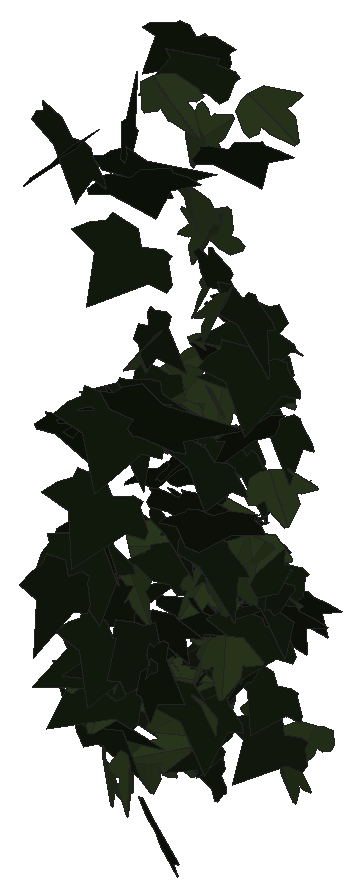
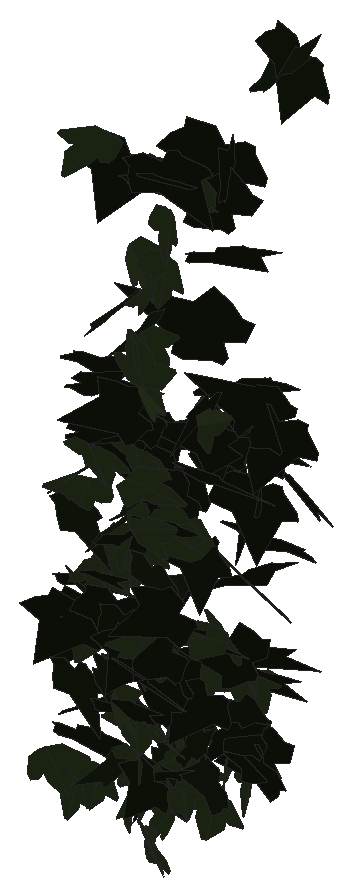
# SketchUp Ruby script. Lengths in inches.
U = 1.inch
M = Sketchup.active_model
def pt(a) = Geom::Point3d.new(a.map { |v| v * U })
def face(e, loops, mat)
  f = e.add_face(loops[0].map { |a| pt(a) })
  loops[1..].each { |l| e.add_face(l.map { |a| pt(a) }).erase! }
  f.material = f.back_material = mat if mat
  f
end
# faces: each face lists its corners as indices into pts; further lists are holes
def faces(e, pts, list, mat = nil) = list.each { |f| face(e, (f[0].is_a?(Array) ? f : [f]).map { |l| l.map { |i| pts[i] } }, mat) }
# xy, xz, yz: faces in a plane at the given z, y or x. An outline is a flat list of corners, or four numbers for a rectangle; further outlines are holes
def ring(l) = l.size == 4 ? [[l[0], l[1]], [l[2], l[1]], [l[2], l[3]], [l[0], l[3]]] : l.each_slice(2).to_a
def flat(e, list, mat, &to3) = list.each { |f| face(e, (f[0].is_a?(Array) ? f : [f]).map { |l| ring(l).map { |u, v| to3.(u, v) } }, mat) }
def xy(e, z, list, mat = nil) = flat(e, list, mat) { |x, y| [x, y, z] }
def xz(e, y, list, mat = nil) = flat(e, list, mat) { |x, z| [x, y, z] }
def yz(e, x, list, mat = nil) = flat(e, list, mat) { |y, z| [x, y, z] }
def lines(e, pts, list) = list.each { |a, b| e.add_line(pt(pts[a]), pt(pts[b])) }
# prism: a flat outline (further loops are holes) pulled along v
def prism(e, loops, v, mat = nil)
  f = face(e, loops, mat); d = Geom::Vector3d.new(v.map { |x| x * U })
  f.pushpull(f.normal.samedirection?(d) ? d.length : -d.length)
end
def box(e, o, s, mat = nil) = prism(e, [[o, [o[0] + s[0], o[1], o[2]], [o[0] + s[0], o[1] + s[1], o[2]], [o[0], o[1] + s[1], o[2]]]], [0, 0, s[2]], mat)
def at(x, y, z, deg = 0) = Geom::Transformation.translation(pt([x, y, z])) * Geom::Transformation.rotation(ORIGIN, Z_AXIS, deg.degrees)
def axes(o, x, y, z) = Geom::Transformation.new([*x, 0, *y, 0, *z, 0, *pt(o).to_a, 1])
def part(name) = M.definitions.add(name)
# library, detail: a bought-in or finely detailed component or shape, given as its bounding box
def library(name, o, s) = part(name).tap { |d| box(d.entities, o, s) }
def detail(e, o, s) = box(e.add_group.entities, o, s)
def put(e, d, t, mat = nil) = e.add_instance(d, t).tap { |i| i.material = mat if mat }
def group(e, t, mat = nil) = e.add_group.tap { |g| g.transformation = t; g.material = mat if mat }.entities
root = M.entities
M.materials.add("1026 AP 7946 SUNNY SIDE UP").color = [254, 231, 186]
M.materials.add("efeu1").color = [18, 25, 13]
M.materials.add("efeu2").color = [43, 57, 29]
c1 = part("ivyleaf_9")
p = [[1.54,2.16,1.25],[1.36,2.04,1.19],[-0.21,0.99,0.68],[-0.71,1.11,0.82],[-0.85,0.86,0.67],[-0.8,0.17,0.21],
  [-0.9,-0.01,0.1],[-0.67,-0.16,-0.02],[-0.08,-0.08,-0.05],[-0.03,-0.6,-0.4],[0.65,-0.88,-0.66],[0.83,-0.6,-0.49],
  [1.29,-0.42,-0.43],[1.8125,-0.07,-0.26],[1.21,0.44,0.15]]
faces(c1.entities,p,[[0,1,2,3,4,5,6,7,8,9,10,11,12,13,14]],"efeu1")
c2 = part("ivyleaf_10")
p = [[0,0.5,-0.03],[-0.0625,2.02,-0.43],[-0.19,2.01,-0.46],[-0.54,1.05,-0.29],[-0.52,0.625,-0.18],[-0.83,0.76,-0.28],
  [-1.16,0.64,-0.33],[-1.15,0.33,-0.24],[-0.77,-0.39,0.02],[-0.3,-0.51,0.16],[0.04,-0.48,0.23],[-0.02,2.01,-0.4375],
  [-0.06,2.01,-0.43],[0.04,-0.49,0.23],[0.67,-0.49,0.14],[1.38,0.36,-0.2],[1.375,0.51,-0.24],[0.81,0.65,-0.19],
  [0.62,0.59,-0.15],[0.6,1.09,-0.28],[0.5,1.23,-0.31]]
faces(c2.entities,p,[[0,1,2,3,4,5,6,7,8,9,10],[11,12,0,13,14,15,16,17,18,19,20]],"efeu2")
put(root,c1,axes([98.38,212.04,285.3],[-0.42534,0.09276,0.15739],[-0.27682,-0.04193,-0.27204],[-0.09708,-0.28684,0.08616]),"1026 AP 7946 SUNNY SIDE UP")
put(root,c1,axes([97.67,211.22,280.16],[-0.05565,-0.06134,-0.33985],[0.53891,0.05005,-0.04487],[0.09666,-0.31438,0.0545]),"1026 AP 7946 SUNNY SIDE UP")
put(root,c1,axes([97.57,211.11,280.16],[0.2723,-0.09417,0.2796],[0.37212,-0.14442,-0.20097],[0.29237,0.27152,-0.0046]),"1026 AP 7946 SUNNY SIDE UP")
put(root,c1,axes([97.9,212.59,280.82],[-0.0867,-0.10997,0.27516],[0.03381,-0.26345,-0.11947],[0.4756,-0.00132,0.05865]),"1026 AP 7946 SUNNY SIDE UP")
put(root,c1,axes([97.82,213.23,282.9],[0.4772,-0.04186,-0.00935],[-0.0204,-0.02537,-0.30326],[0.06947,0.28008,-0.02484]),"1026 AP 7946 SUNNY SIDE UP")
put(root,c2,axes([97.74,212.82,284.58],[-0.21631,-0.05215,0.29035],[0.38492,0.15206,0.14712],[-0.26962,0.25892,-0.02291]),"1026 AP 7946 SUNNY SIDE UP")
put(root,c1,axes([98.28,212.81,290.96],[0.17054,0.12703,-0.30451],[-0.26676,-0.23939,-0.17622],[-0.45956,0.1861,-0.01071]),"1026 AP 7946 SUNNY SIDE UP")
put(root,c1,axes([97.82,211.32,281.89],[0.05548,0.0684,0.35201],[0.47133,0.17878,-0.06705],[-0.3181,0.27683,-0.03796]),"1026 AP 7946 SUNNY SIDE UP")
put(root,c1,axes([98.17,212.1,284.02],[0.11313,0.29038,-0.01214],[0.00712,-0.01647,-0.31908],[-0.49355,0.06632,-0.00739]),"1026 AP 7946 SUNNY SIDE UP")
put(root,c1,axes([98.08,211.8,279.93],[-0.09047,0.25353,-0.13791],[-0.12801,0.11717,0.27492],[0.46813,0.08104,0.04852]),"1026 AP 7946 SUNNY SIDE UP")
put(root,c2,axes([98.42,213.16,284.79],[-0.2338,0.04398,-0.27004],[-0.35977,0.14226,0.15209],[0.24559,0.25028,-0.03427]),"1026 AP 7946 SUNNY SIDE UP")
put(root,c1,axes([98.05,210.36,285.49],[0.49043,0.19126,-0.1099],[-0.12411,-0.07954,-0.37108],[-0.34909,0.29697,-0.02246]),"1026 AP 7946 SUNNY SIDE UP")
put(root,c2,axes([97.74,212.98,285.03],[0.2767,0.02598,0.27299],[0.4345,-0.01331,-0.17413],[-0.00466,0.30206,-0.02689]),"1026 AP 7946 SUNNY SIDE UP")
put(root,c1,axes([97.94,211.39,280.71],[0.06599,-0.21099,-0.23244],[-0.0259,0.21449,-0.22598],[0.50994,0.0382,0.0186]),"1026 AP 7946 SUNNY SIDE UP")
put(root,c1,axes([97.86,213.04,283.46],[0.38777,0.11533,0.1459],[0.2122,0.05124,-0.27306],[-0.21364,0.26023,-0.00641]),"1026 AP 7946 SUNNY SIDE UP")
put(root,c1,axes([98.22,213.09,284.92],[-0.45097,-0.12442,-0.02544],[0.06144,-0.02551,-0.31172],[0.20555,-0.26536,0.03735]),"1026 AP 7946 SUNNY SIDE UP")
put(root,c1,axes([97.89,211.09,280.59],[0.1587,0.29361,-0.07654],[0.0097,0.0771,0.33043],[0.51447,-0.09203,0.01738]),"1026 AP 7946 SUNNY SIDE UP")
put(root,c2,axes([98.1875,211.97,286.16],[-0.10391,0.08457,-0.30816],[-0.14064,-0.28821,-0.07554],[-0.49134,0.06461,0.08679]),"1026 AP 7946 SUNNY SIDE UP")
put(root,c1,axes([98.4,210.71,281.51],[-0.43874,-0.14077,0.19038],[-0.2317,-0.12222,-0.31443],[0.31054,-0.29007,0.03437]),"1026 AP 7946 SUNNY SIDE UP")
put(root,c2,axes([98.24,210.84,279.62],[-0.30541,0.25759,0.06524],[-0.11552,0.02207,-0.33298],[-0.43291,-0.18761,0.04283]),"1026 AP 7946 SUNNY SIDE UP")
put(root,c2,axes([98.12,213.28,289.1],[0.1476,-0.01866,-0.31434],[0.11735,0.29866,0.00577],[0.48503,-0.06658,0.09426]),"1026 AP 7946 SUNNY SIDE UP")
put(root,c2,axes([98.41,213.26,285.63],[0.20047,0.11119,-0.25724],[-0.36063,-0.11983,-0.17179],[-0.27195,0.24087,0.03819]),"1026 AP 7946 SUNNY SIDE UP")
put(root,c2,axes([97.86,212.15,282.62],[0.11133,-0.03432,-0.30863],[0.4711,0.09268,0.05716],[0.14214,-0.28029,0.05229]),"1026 AP 7946 SUNNY SIDE UP")
put(root,c1,axes([98.09,212.06,281.53],[0.48351,0.07693,-0.06155],[-0.08092,-0.04655,-0.31466],[-0.14272,0.28702,-0.03013]),"1026 AP 7946 SUNNY SIDE UP")
put(root,c1,axes([98.21,213.17,280.51],[0.13488,0.21504,0.17202],[0.11905,0.1421,-0.24302],[-0.43693,0.1051,-0.01311]),"1026 AP 7946 SUNNY SIDE UP")
put(root,c2,axes([98.26,211.66,279.46],[-0.48743,0.0251,-0.01062],[0.01287,-0.03031,-0.30738],[-0.04419,-0.28572,0.02761]),"1026 AP 7946 SUNNY SIDE UP")
put(root,c1,axes([98.18,211.9,286.48],[0.17429,-0.15766,-0.26731],[-0.22103,0.21067,-0.19845],[0.44664,0.16578,0.0061]),"1026 AP 7946 SUNNY SIDE UP")
put(root,c2,axes([98.41,211.76,280.7],[0.19147,-0.02456,0.28268],[-0.28092,0.21811,0.10032],[-0.35244,-0.18719,0.0736]),"1026 AP 7946 SUNNY SIDE UP")
put(root,c1,axes([98.62,212.22,282.52],[-0.41568,-0.0099,0.16834],[-0.26152,-0.04691,-0.26046],[0.05703,-0.28728,0.0326]),"1026 AP 7946 SUNNY SIDE UP")
put(root,c2,axes([98.28,213.125,279.41],[0.208,-0.23771,0.07003],[0.04232,-0.0642,-0.2871],[0.41781,0.12484,-0.00578]),"1026 AP 7946 SUNNY SIDE UP")
put(root,c2,axes([98.04,211.61,282.33],[0.30397,-0.06339,0.24508],[0.35983,-0.08901,-0.20441],[0.18495,0.27736,-0.00511]),"1026 AP 7946 SUNNY SIDE UP")
put(root,c1,axes([98.53,210.64,281.14],[-0.52435,-0.14158,0.07959],[-0.07607,-0.08265,-0.36011],[0.2621,-0.30722,0.0547]),"1026 AP 7946 SUNNY SIDE UP")
put(root,c1,axes([98.6,212.85,290.6],[-0.51653,-0.07383,0.09281],[-0.12357,-0.06758,-0.3324],[0.15026,-0.30936,0.0457]),"1026 AP 7946 SUNNY SIDE UP")
put(root,c2,axes([98.52,210.6,281.59],[0.20623,-0.15301,-0.30995],[-0.20112,0.26508,-0.20092],[0.515,0.16479,0.04565]),"1026 AP 7946 SUNNY SIDE UP")
put(root,c1,axes([98.4,211.12,289.92],[-0.00384,-0.13812,0.34401],[0.19076,0.30589,0.14508],[-0.56521,0.10418,0.04663]),"1026 AP 7946 SUNNY SIDE UP")
put(root,c2,axes([98.31,213.03,282.66],[0.45847,0.10416,-0.01682],[-0.00974,-0.03233,-0.30889],[-0.17891,0.26868,-0.02628]),"1026 AP 7946 SUNNY SIDE UP")
put(root,c2,axes([98.32,212.29,279.87],[0.23425,0.23714,-0.06842],[-0.03202,-0.0664,-0.29412],[-0.41709,0.13828,-0.01584]),"1026 AP 7946 SUNNY SIDE UP")
put(root,c2,axes([98.34,213.22,287.49],[-0.4877,0.03191,0.09177],[0.14907,0.02219,0.30805],[0.04101,0.29887,-0.02843]),"1026 AP 7946 SUNNY SIDE UP")
put(root,c2,axes([98.46,212.96,287.87],[-0.06737,-0.3227,0.0988],[0.01143,-0.09938,-0.33534],[0.53005,-0.03887,0.01979]),"1026 AP 7946 SUNNY SIDE UP")
put(root,c2,axes([98.39,210.67,281.11],[0.43977,0.21061,-0.10946],[-0.10718,-0.08822,-0.35747],[-0.38483,0.26524,-0.02553]),"1026 AP 7946 SUNNY SIDE UP")
put(root,c1,axes([98.72,213.31,282.39],[-0.43052,0.10167,0.06437],[-0.11368,-0.01021,-0.29044],[-0.1638,-0.26014,0.03237]),"1026 AP 7946 SUNNY SIDE UP")
put(root,c2,axes([98.22,213.11,279.34],[0.2994,-0.10835,0.18852],[0.24511,-0.10371,-0.22281],[0.25408,0.22773,-0.00721]),"1026 AP 7946 SUNNY SIDE UP")
put(root,c1,axes([98.5,212.95,280.39],[-0.32283,-0.20437,0.11645],[-0.05361,-0.12417,-0.2928],[0.36419,-0.19944,0.06012]),"1026 AP 7946 SUNNY SIDE UP")
put(root,c1,axes([98.51,210.26,284.12],[0.21313,0.32211,-0.05701],[-0.0203,-0.05698,-0.37077],[-0.55505,0.12577,-0.00833]),"1026 AP 7946 SUNNY SIDE UP")
put(root,c2,axes([98.54,212.42,289.73],[-0.37473,0.22786,0.05808],[-0.12453,-0.00065,-0.33498],[-0.37641,-0.22663,0.053]),"1026 AP 7946 SUNNY SIDE UP")
put(root,c1,axes([98.2,211.39,285.23],[0.45531,-0.14709,-0.11456],[0.18635,-0.01687,0.32499],[-0.24382,-0.28758,0.03445]),"1026 AP 7946 SUNNY SIDE UP")
put(root,c1,axes([98.27,210.34,283.46],[-0.31164,-0.22997,-0.19067],[0.37138,0.02503,-0.28039],[0.32069,-0.25246,0.13941]),"1026 AP 7946 SUNNY SIDE UP")
put(root,c1,axes([98.12,210.33,285.53],[0.28297,0.29373,-0.14645],[0.09611,0.12943,0.36309],[0.5444,-0.17553,0.01202]),"1026 AP 7946 SUNNY SIDE UP")
put(root,c1,axes([98.16,212.82,281.62],[0.1178,-0.1221,0.2741],[0.1923,-0.23151,-0.15337],[0.44412,0.13263,-0.0063]),"1026 AP 7946 SUNNY SIDE UP")
put(root,c2,axes([98.35,213.24,282.87],[0.2391,0.23915,0.07251],[0.06589,0.05211,-0.29631],[-0.41533,0.14594,-0.00526]),"1026 AP 7946 SUNNY SIDE UP")
put(root,c1,axes([98.32,212.99,282.71],[0.39271,-0.16709,-0.05986],[0.09449,-0.01447,0.30452],[-0.28256,-0.23706,0.01864]),"1026 AP 7946 SUNNY SIDE UP")
put(root,c2,axes([98.34,212.32,280.51],[0.01689,-0.12217,-0.267],[0.25699,0.20984,-0.10132],[0.39233,-0.13219,0.07786]),"1026 AP 7946 SUNNY SIDE UP")
put(root,c2,axes([98.26,212.125,290.41],[-0.38461,-0.02647,-0.24911],[0.35217,-0.17203,-0.198],[-0.18317,-0.27517,0.14237]),"1026 AP 7946 SUNNY SIDE UP")
put(root,c1,axes([98.7,212.31,280.49],[-0.30423,0.13392,-0.18748],[0.14679,-0.16721,-0.23169],[-0.34681,-0.18825,0.0664]),"1026 AP 7946 SUNNY SIDE UP")
put(root,c1,axes([98.5,213.15,282.7],[0.28473,0.2217,0.06273],[0.06257,0.04195,-0.297],[-0.38296,0.17168,-0.00189]),"1026 AP 7946 SUNNY SIDE UP")
put(root,c2,axes([98.53,212.91,287.03],[0.14309,-0.23347,0.19898],[0.09232,-0.18109,-0.26812],[0.50137,0.09997,-0.00742]),"1026 AP 7946 SUNNY SIDE UP")
put(root,c2,axes([98.6,213.2,280.08],[-0.07307,0.26811,-0.0087],[-0.07757,-0.01892,-0.28639],[-0.44891,-0.04037,0.0509]),"1026 AP 7946 SUNNY SIDE UP")
put(root,c1,axes([98.41,211.15,285.28],[0.04289,-0.32652,0.0938],[0.02275,-0.09201,-0.33802],[0.53332,0.03018,0.00687]),"1026 AP 7946 SUNNY SIDE UP")
put(root,c2,axes([98.59,213.18,280.74],[-0.31855,0.18368,-0.08246],[0.06297,-0.07506,-0.28073],[-0.33381,-0.18944,0.02573]),"1026 AP 7946 SUNNY SIDE UP")
put(root,c1,axes([98.69,210.12,284],[0.33784,-0.10921,-0.31594],[-0.4433,0.13446,-0.24111],[0.29395,0.3283,-0.00049]),"1026 AP 7946 SUNNY SIDE UP")
put(root,c1,axes([98.75,210.92,288.4375],[-0.4525,-0.25432,0.08779],[-0.0413,-0.09686,-0.39184],[0.45348,-0.26259,0.05191]),"1026 AP 7946 SUNNY SIDE UP")
put(root,c2,axes([98.69,212.23,279.35],[0.05386,0.09117,0.27613],[-0.12049,0.25231,-0.08301],[-0.44651,-0.05709,0.05571]),"1026 AP 7946 SUNNY SIDE UP")
put(root,c1,axes([98.22,211.41,285.53],[0.23928,-0.00573,-0.30735],[0.36725,0.21228,0.11218],[0.3203,-0.23912,0.10098]),"1026 AP 7946 SUNNY SIDE UP")
put(root,c2,axes([98.82,211.71,279.73],[-0.09609,0.00333,0.31322],[-0.11336,-0.29024,-0.01434],[0.48351,-0.06738,0.05888]),"1026 AP 7946 SUNNY SIDE UP")
put(root,c2,axes([98.54,210.9,279.68],[-0.00827,-0.23092,0.23454],[0.27641,-0.19307,-0.2138],[0.4684,0.10986,0.1303]),"1026 AP 7946 SUNNY SIDE UP")
put(root,c1,axes([98.46,212.03,283.21],[0.0747,-0.25477,0.15485],[0.0887,-0.14048,-0.27757],[0.49221,0.06398,0.02652]),"1026 AP 7946 SUNNY SIDE UP")
put(root,c2,axes([98.66,212.7,279.91],[-0.1836,0.24466,-0.0332],[0.00883,-0.03507,-0.28669],[-0.41927,-0.10787,0.0085]),"1026 AP 7946 SUNNY SIDE UP")
put(root,c2,axes([98.77,212.2,288.77],[-0.46182,0.16568,0.03144],[-0.06374,-0.00954,-0.33987],[-0.2778,-0.27324,0.02571]),"1026 AP 7946 SUNNY SIDE UP")
put(root,c1,axes([98.85,208.79,290.84],[0.11746,0.35288,0.21928],[0.08673,0.19392,-0.38209],[-0.68326,0.08528,-0.0108]),"1026 AP 7946 SUNNY SIDE UP")
put(root,c2,axes([98.96,211.71,280.55],[0.06525,-0.0099,-0.34831],[-0.19498,0.30598,-0.02024],[0.51676,0.1167,0.03634]),"1026 AP 7946 SUNNY SIDE UP")
put(root,c1,axes([98.92,213.18,281.59],[-0.43267,-0.10773,0.02606],[-0.02329,-0.03339,-0.29547],[0.18658,-0.25399,0.02355]),"1026 AP 7946 SUNNY SIDE UP")
put(root,c1,axes([99.13,212.55,282.5],[-0.3457,0.05056,0.21516],[-0.34455,-0.10143,-0.19492],[0.06542,-0.26704,0.11037]),"1026 AP 7946 SUNNY SIDE UP")
put(root,c2,axes([98.6,211.25,281.51],[-0.2243,0.18536,-0.2502],[0.18659,-0.21019,-0.24544],[-0.47419,-0.17039,0.02177]),"1026 AP 7946 SUNNY SIDE UP")
put(root,c1,axes([98.97,212.21,283.47],[-0.07676,0.28787,0.07099],[-0.01841,0.06162,-0.31111],[-0.49974,-0.04649,0.00055]),"1026 AP 7946 SUNNY SIDE UP")
put(root,c1,axes([98.93,212.91,282.95],[0.00231,0.28144,-0.03927],[-0.00121,-0.04034,-0.30187],[-0.48263,0.00145,0.00057]),"1026 AP 7946 SUNNY SIDE UP")
put(root,c1,axes([98.35,211.17,289.41],[0.1069,-0.07156,0.35066],[0.56176,-0.04569,-0.07921],[0.10055,0.33132,0.06975]),"1026 AP 7946 SUNNY SIDE UP")
put(root,c2,axes([98.76,212.49,285.34],[-0.32658,0.22506,-0.06435],[0.04129,-0.06193,-0.31702],[-0.39459,-0.19275,0.02009]),"1026 AP 7946 SUNNY SIDE UP")
put(root,c1,axes([98.8,211.62,284.53],[0.10474,0.20282,0.26138],[0.17639,0.21927,-0.2225],[-0.50546,0.11854,-0.02348]),"1026 AP 7946 SUNNY SIDE UP")
put(root,c1,axes([99,212.375,280.08],[-0.23493,0.19189,-0.15304],[0.08957,-0.13952,-0.25275],[-0.39881,-0.14438,0.03338]),"1026 AP 7946 SUNNY SIDE UP")
put(root,c2,axes([98.99,211.71,280.39],[-0.22722,0.23274,0.21149],[-0.22393,0.14678,-0.28316],[-0.46365,-0.18495,0.03312]),"1026 AP 7946 SUNNY SIDE UP")
put(root,c1,axes([98.875,209.07,283.74],[-0.52867,0.01157,-0.26663],[0.40822,-0.09217,-0.3276],[-0.11272,-0.38807,0.06413]),"1026 AP 7946 SUNNY SIDE UP")
put(root,c1,axes([98.86,210.36,285.88],[-0.38672,-0.31054,-0.01106],[0.04292,-0.01078,-0.41148],[0.52551,-0.22764,0.02547]),"1026 AP 7946 SUNNY SIDE UP")
put(root,c2,axes([98.92,212.24,282.3],[0.16415,0.18631,-0.21608],[-0.14589,-0.18542,-0.22721],[-0.44607,0.12921,-0.0052]),"1026 AP 7946 SUNNY SIDE UP")
put(root,c2,axes([98.83,213,284.35],[-0.04569,0.29079,-0.06829],[-0.00018,-0.06786,-0.31353],[-0.50679,-0.02619,0.00627]),"1026 AP 7946 SUNNY SIDE UP")
put(root,c1,axes([98.95,209.99,284.71],[-0.54936,-0.17117,-0.08988],[0.16824,-0.01479,-0.3872],[0.27454,-0.33345,0.05743]),"1026 AP 7946 SUNNY SIDE UP")
put(root,c1,axes([98.88,212.97,284.4375],[-0.27014,-0.25328,0.01585],[0.00556,-0.02341,-0.32015],[0.43102,-0.15844,0.01406]),"1026 AP 7946 SUNNY SIDE UP")
put(root,c2,axes([98.82,212.81,281.14],[0.46491,0.02676,0.01568],[0.02535,-0.0058,-0.29458],[-0.04483,0.27418,-0.0039]),"1026 AP 7946 SUNNY SIDE UP")
put(root,c2,axes([98.93,213.02,281.58],[0.03659,-0.27424,0.08401],[0.01973,-0.08137,-0.29559],[0.48552,0.02397,0.00568]),"1026 AP 7946 SUNNY SIDE UP")
put(root,c1,axes([98.5,212.1,281.7],[0.26622,-0.0348,0.25658],[0.39068,-0.0692,-0.17262],[0.13043,0.27832,-0.00665]),"1026 AP 7946 SUNNY SIDE UP")
put(root,c1,axes([98.71,209.41,290.9],[-0.05427,-0.32475,0.27647],[0.0601,-0.2644,-0.3493],[0.70627,-0.00246,0.05097]),"1026 AP 7946 SUNNY SIDE UP")
put(root,c1,axes([99.24,212.54,281.14],[-0.40944,0.14535,0.04689],[-0.08321,-0.00049,-0.30026],[-0.24294,-0.24481,0.02382]),"1026 AP 7946 SUNNY SIDE UP")
put(root,c1,axes([98.82,213.19,280.59],[0.30677,-0.20202,-0.03912],[-0.00911,0.04053,-0.28859],[0.34762,0.17935,0.02696]),"1026 AP 7946 SUNNY SIDE UP")
put(root,c1,axes([99.02,209.95,282.38],[-0.25456,-0.31787,0.09025],[-0.02598,-0.09035,-0.37666],[0.5595,-0.14882,0.02357]),"1026 AP 7946 SUNNY SIDE UP")
put(root,c1,axes([99.05,210.41,289.93],[0.38496,0.32402,-0.03783],[-0.00588,-0.04578,-0.42331],[-0.55408,0.2256,-0.02179]),"1026 AP 7946 SUNNY SIDE UP")
put(root,c2,axes([99.18,212.53,282.22],[0.26416,-0.21956,-0.11763],[-0.10803,0.08606,-0.2869],[0.40031,0.16811,0.0002]),"1026 AP 7946 SUNNY SIDE UP")
put(root,c1,axes([98.75,212.93,286.57],[0.47653,-0.04377,0.12915],[0.19934,-0.03276,-0.3043],[0.09008,0.30401,-0.00982]),"1026 AP 7946 SUNNY SIDE UP")
put(root,c1,axes([99.22,212.22,279.21],[-0.10878,0.00513,0.29301],[-0.18657,-0.25786,-0.02598],[0.42547,-0.11176,0.06352]),"1026 AP 7946 SUNNY SIDE UP")
put(root,c1,axes([98.96,212.35,287.67],[0.26026,-0.2706,-0.05007],[-0.05533,0.03119,-0.33225],[0.46189,0.15621,-0.01159]),"1026 AP 7946 SUNNY SIDE UP")
put(root,c2,axes([99.08,212.38,285.49],[0.49856,-0.0535,0.05721],[0.08189,-0.0361,-0.31885],[0.09995,0.29646,-0.02416]),"1026 AP 7946 SUNNY SIDE UP")
put(root,c2,axes([99.22,211.99,281.42],[0.2243,-0.24776,0.09603],[0.04225,-0.09177,-0.30111],[0.4472,0.13294,-0.01972]),"1026 AP 7946 SUNNY SIDE UP")
put(root,c1,axes([99.28,212.6875,282.99],[0.28865,0.21153,-0.10844],[-0.08012,-0.09515,-0.29099],[-0.39208,0.17518,-0.02038]),"1026 AP 7946 SUNNY SIDE UP")
put(root,c1,axes([99.01,212.27,286.16],[0.50663,-0.06743,0.00278],[-0.00527,-0.02944,-0.32646],[0.1145,0.29701,-0.02733]),"1026 AP 7946 SUNNY SIDE UP")
put(root,c1,axes([99.75,209.77,282.48],[-0.5417,0.21442,0.02803],[-0.06285,-0.01331,-0.41038],[-0.36071,-0.31969,0.02941]),"1026 AP 7946 SUNNY SIDE UP")
put(root,c2,axes([99.65,211.02,281],[0.47994,-0.02876,-0.2137],[-0.32698,0.06113,-0.30122],[0.09925,0.34043,0.04098]),"1026 AP 7946 SUNNY SIDE UP")
put(root,c1,axes([99.29,212.79,284.28],[0.09147,-0.28743,0.04889],[0.00048,-0.0502,-0.31364],[0.49509,0.05315,-0.00873]),"1026 AP 7946 SUNNY SIDE UP")
put(root,c2,axes([99.54,212.84,280.02],[-0.43079,0.11108,-0.00629],[-0.00593,-0.02617,-0.29569],[-0.18887,-0.25253,0.02363]),"1026 AP 7946 SUNNY SIDE UP")
put(root,c1,axes([99.86,212.72,286.61],[-0.36953,-0.0703,0.21768],[-0.3023,-0.1057,-0.24363],[0.20752,-0.27916,0.03272]),"1026 AP 7946 SUNNY SIDE UP")
put(root,c2,axes([99.53,212.9,285.61],[0.50948,-0.03926,-0.00533],[-0.01348,-0.02645,-0.3231],[0.06571,0.29899,-0.025]),"1026 AP 7946 SUNNY SIDE UP")
put(root,c1,axes([99.89,212.76,285.78],[-0.31204,-0.03483,0.25451],[-0.35645,-0.12334,-0.19452],[0.19981,-0.27442,0.05046]),"1026 AP 7946 SUNNY SIDE UP")
put(root,c1,axes([99.48,211.02,284.4375],[0.5417,0.14307,-0.06342],[-0.06973,-0.05701,-0.37334],[-0.25471,0.31987,-0.03267]),"1026 AP 7946 SUNNY SIDE UP")
put(root,c1,axes([99.93,211.32,280.3125],[-0.3579,0.25438,-0.04321],[0.0231,-0.04536,-0.3538],[-0.43753,-0.21047,0.01667]),"1026 AP 7946 SUNNY SIDE UP")
put(root,c2,axes([99.93,212.21,283.23],[-0.17605,-0.23991,0.20278],[0.00331,-0.2037,-0.27344],[0.52218,-0.07959,0.0701]),"1026 AP 7946 SUNNY SIDE UP")
put(root,c1,axes([100.03,212.03,285.42],[-0.0951,0.25459,-0.22404],[0.06339,-0.20938,-0.28191],[-0.55945,-0.067,0.00614]),"1026 AP 7946 SUNNY SIDE UP")
put(root,c1,axes([99.95,212.23,281.38],[-0.32026,0.13127,-0.22133],[0.24387,-0.15466,-0.24563],[-0.3397,-0.23479,0.03233]),"1026 AP 7946 SUNNY SIDE UP")
put(root,c1,axes([99.81,211.74,290.08],[0.40681,0.264,-0.01654],[0.00787,-0.02967,-0.38131],[-0.44923,0.23855,-0.02166]),"1026 AP 7946 SUNNY SIDE UP")
put(root,c2,axes([99.98,211.35,283.25],[-0.56954,0.09118,0.04258],[-0.08207,-0.03191,-0.36978],[-0.14668,-0.33621,0.04156]),"1026 AP 7946 SUNNY SIDE UP")
put(root,c1,axes([100.07,212.69,281.53],[-0.0849,0.29672,-0.01758],[0.00289,-0.02029,-0.32242],[-0.50487,-0.05001,0.00111]),"1026 AP 7946 SUNNY SIDE UP")
put(root,c1,axes([99.81,211.12,281.12],[-0.16888,-0.32266,-0.0233],[0.03034,0.01284,-0.36102],[0.5477,-0.1002,0.01282]),"1026 AP 7946 SUNNY SIDE UP")
put(root,c1,axes([99.97,209.68,282.35],[0.17224,-0.10399,-0.39545],[-0.40618,0.27977,-0.15135],[0.50644,0.25975,0.01311]),"1026 AP 7946 SUNNY SIDE UP")
put(root,c2,axes([99.96,212.25,283.27],[0.16947,0.29766,-0.0822],[-0.10047,-0.06471,-0.335],[-0.51379,0.11084,0.0384]),"1026 AP 7946 SUNNY SIDE UP")
put(root,c1,axes([99.85,211.28,285.0625],[-0.19363,-0.28008,0.15393],[0.12755,-0.18421,-0.2849],[0.4838,-0.06353,0.13672]),"1026 AP 7946 SUNNY SIDE UP")
put(root,c2,axes([99.87,212.3,282.22],[0.31849,0.20777,0.168],[0.07465,0.16211,-0.28885],[-0.43285,0.18084,0.0738]),"1026 AP 7946 SUNNY SIDE UP")
put(root,c1,axes([99.74,210.1,279.36],[0.06299,-0.13535,0.35907],[0.10522,-0.33159,-0.15444],[0.6077,0.07144,-0.01048]),"1026 AP 7946 SUNNY SIDE UP")
put(root,c1,axes([100.07,212.1875,281.98],[-0.36063,-0.23386,0.01954],[0.00157,-0.02955,-0.33795],[0.39863,-0.21145,0.019]),"1026 AP 7946 SUNNY SIDE UP")
put(root,c2,axes([100,211.41,281.94],[0.21843,0.31011,-0.06848],[-0.07469,-0.05526,-0.35963],[-0.53373,0.13465,0.0223]),"1026 AP 7946 SUNNY SIDE UP")
put(root,c2,axes([99.87,212.35,290.6],[0.22397,0.24351,0.22309],[0.12376,0.19313,-0.29284],[-0.52623,0.14906,0.02608]),"1026 AP 7946 SUNNY SIDE UP")
put(root,c1,axes([99.51,209.95,286.27],[0.1706,-0.0393,0.40776],[0.61922,-0.11163,-0.11678],[0.20046,0.37828,0.0137]),"1026 AP 7946 SUNNY SIDE UP")
put(root,c1,axes([99.89,212.9,285.09],[-0.01368,-0.31898,0.08898],[0.0135,-0.0884,-0.32907],[0.5202,-0.00609,0.01088]),"1026 AP 7946 SUNNY SIDE UP")
put(root,c1,axes([100.23,212.4,283.01],[-0.44144,-0.14905,0.0777],[-0.07209,-0.07429,-0.31875],[0.27355,-0.26011,0.04139]),"1026 AP 7946 SUNNY SIDE UP")
put(root,c2,axes([100.14,211.11,287.98],[0.03396,-0.34706,0.05644],[0.00181,-0.05679,-0.35856],[0.55297,0.0215,-0.00229]),"1026 AP 7946 SUNNY SIDE UP")
put(root,c1,axes([100.08,212.46,280.87],[-0.2293,-0.24187,0.1262],[-0.01871,-0.13025,-0.29365],[0.45874,-0.12621,0.0511]),"1026 AP 7946 SUNNY SIDE UP")
put(root,c1,axes([99.89,211.95,287.48],[0.10868,-0.33432,0.03177],[-0.00022,-0.03468,-0.36484],[0.57046,0.06368,-0.00619]),"1026 AP 7946 SUNNY SIDE UP")
put(root,c1,axes([100.35,212.26,282.79],[-0.45694,0.15215,-0.08999],[0.09652,-0.07317,-0.32999],[-0.28059,-0.27296,0.03303]),"1026 AP 7946 SUNNY SIDE UP")
put(root,c2,axes([100.18,212.6,279.57],[-0.41541,0.1676,0.01879],[-0.04503,-0.01164,-0.31661],[-0.28214,-0.24492,0.02287]),"1026 AP 7946 SUNNY SIDE UP")
put(root,c1,axes([100.375,212.36,284.17],[-0.18375,0.28472,-0.07783],[0.02813,-0.07539,-0.32694],[-0.49964,-0.10895,0.01021]),"1026 AP 7946 SUNNY SIDE UP")
put(root,c1,axes([100.34,212.26,280.23],[-0.49407,-0.10548,-0.0209],[0.04212,-0.01536,-0.33074],[0.17674,-0.29121,0.0204]),"1026 AP 7946 SUNNY SIDE UP")
put(root,c1,axes([99.97,211.09,283.79],[0.02246,-0.34807,0.05632],[0.07655,-0.05505,-0.3709],[0.59386,0.02026,0.04568]),"1026 AP 7946 SUNNY SIDE UP")
put(root,c1,axes([100.19,211.91,286.55],[-0.3837,-0.24538,-0.0889],[0.17267,0.01282,-0.35028],[0.40256,-0.23937,0.06551]),"1026 AP 7946 SUNNY SIDE UP")
put(root,c1,axes([100.17,212.21,282.28],[0.4664,0.15993,-0.04047],[-0.03536,-0.04323,-0.33975],[-0.27756,0.27424,-0.02473]),"1026 AP 7946 SUNNY SIDE UP")
put(root,c2,axes([100.4,212.88,280.03],[-0.28286,-0.23297,0.10861],[-0.02048,-0.12194,-0.2975],[0.40243,-0.16996,0.0612]),"1026 AP 7946 SUNNY SIDE UP")
put(root,c1,axes([100.15,212.34,282.53],[0.00978,-0.30071,0.0596],[0.00241,-0.05957,-0.32282],[0.52039,0.00593,0.00038]),"1026 AP 7946 SUNNY SIDE UP")
put(root,c1,axes([100.47,210.51,284.71],[0.21686,0.29908,-0.18548],[-0.13908,-0.15751,-0.35015],[-0.57347,0.1513,0.01478]),"1026 AP 7946 SUNNY SIDE UP")
put(root,c2,axes([100.24,212.21,284.47],[0.33137,0.24391,0.08281],[0.02514,0.08241,-0.33071],[-0.43204,0.19187,0.04427]),"1026 AP 7946 SUNNY SIDE UP")
put(root,c1,axes([100.21,212.53,282.38],[0.4534,0.14734,-0.01057],[0.0006,-0.025,-0.32606],[-0.25091,0.26618,-0.01988]),"1026 AP 7946 SUNNY SIDE UP")
